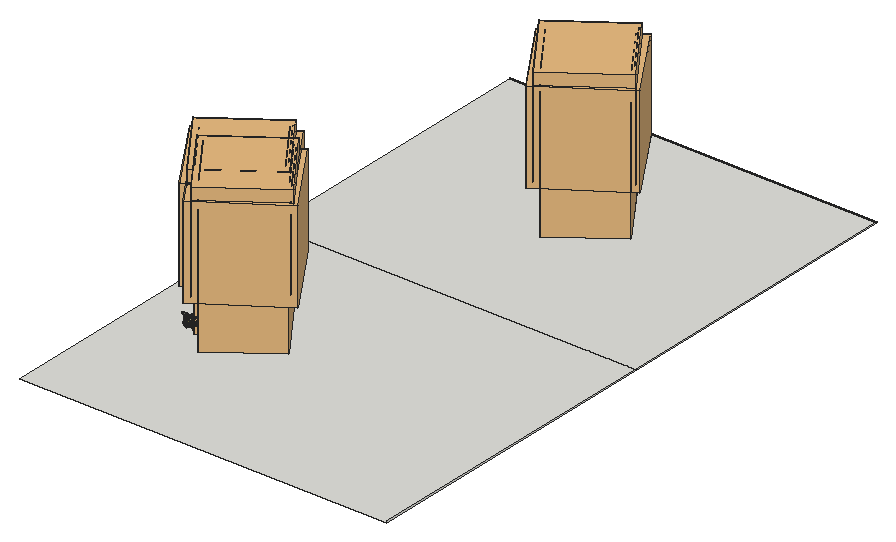
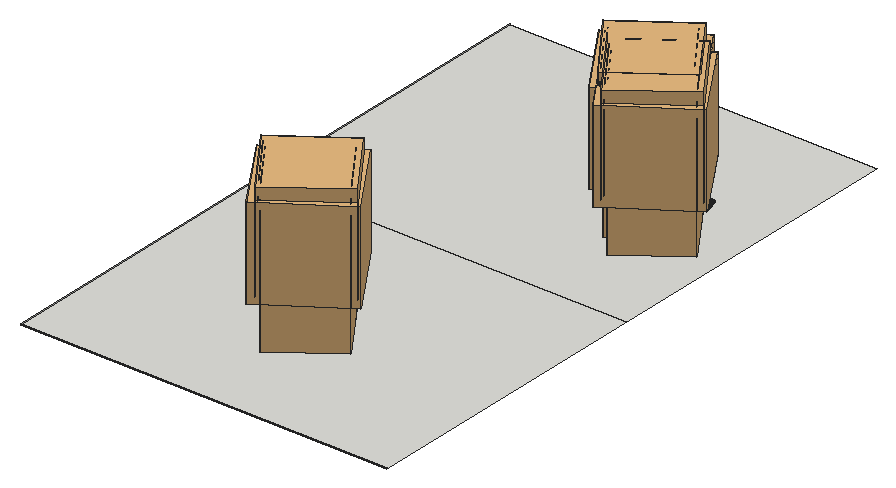
# SketchUp Ruby script. Lengths in inches.
U = 1.inch
M = Sketchup.active_model
def pt(a) = Geom::Point3d.new(a.map { |v| v * U })
def face(e, loops, mat)
  f = e.add_face(loops[0].map { |a| pt(a) })
  loops[1..].each { |l| e.add_face(l.map { |a| pt(a) }).erase! }
  f.material = f.back_material = mat if mat
  f
end
# faces: each face lists its corners as indices into pts; further lists are holes
def faces(e, pts, list, mat = nil) = list.each { |f| face(e, (f[0].is_a?(Array) ? f : [f]).map { |l| l.map { |i| pts[i] } }, mat) }
# xy, xz, yz: faces in a plane at the given z, y or x. An outline is a flat list of corners, or four numbers for a rectangle; further outlines are holes
def ring(l) = l.size == 4 ? [[l[0], l[1]], [l[2], l[1]], [l[2], l[3]], [l[0], l[3]]] : l.each_slice(2).to_a
def flat(e, list, mat, &to3) = list.each { |f| face(e, (f[0].is_a?(Array) ? f : [f]).map { |l| ring(l).map { |u, v| to3.(u, v) } }, mat) }
def xy(e, z, list, mat = nil) = flat(e, list, mat) { |x, y| [x, y, z] }
def xz(e, y, list, mat = nil) = flat(e, list, mat) { |x, z| [x, y, z] }
def yz(e, x, list, mat = nil) = flat(e, list, mat) { |y, z| [x, y, z] }
def lines(e, pts, list) = list.each { |a, b| e.add_line(pt(pts[a]), pt(pts[b])) }
# prism: a flat outline (further loops are holes) pulled along v
def prism(e, loops, v, mat = nil)
  f = face(e, loops, mat); d = Geom::Vector3d.new(v.map { |x| x * U })
  f.pushpull(f.normal.samedirection?(d) ? d.length : -d.length)
end
def box(e, o, s, mat = nil) = prism(e, [[o, [o[0] + s[0], o[1], o[2]], [o[0] + s[0], o[1] + s[1], o[2]], [o[0], o[1] + s[1], o[2]]]], [0, 0, s[2]], mat)
def at(x, y, z, deg = 0) = Geom::Transformation.translation(pt([x, y, z])) * Geom::Transformation.rotation(ORIGIN, Z_AXIS, deg.degrees)
def axes(o, x, y, z) = Geom::Transformation.new([*x, 0, *y, 0, *z, 0, *pt(o).to_a, 1])
def part(name) = M.definitions.add(name)
# library, detail: a bought-in or finely detailed component or shape, given as its bounding box
def library(name, o, s) = part(name).tap { |d| box(d.entities, o, s) }
def detail(e, o, s) = box(e.add_group.entities, o, s)
def put(e, d, t, mat = nil) = e.add_instance(d, t).tap { |i| i.material = mat if mat }
def group(e, t, mat = nil) = e.add_group.tap { |g| g.transformation = t; g.material = mat if mat }.entities
root = M.entities
M.materials.add("028_190k_fullGeometry_Material \#4").color = [120, 148, 64]
M.materials.add("Colorsadfasdfa0sd1f06w3").color = [153, 130, 61]
M.materials.add("Euphorbia asdfasd0f150160s159w").color = [180, 173, 131]
M.materials.add("Euphorbiaasdfa0sdf1a56sd016wow Leaf SU").color = [141, 134, 72]
M.materials.add("asdfasdf0165f6asdLeafVar1sfd015as60f1as6").color = [231, 235, 211]
M.materials.add("dw_stemssadfasdfa0sdf1s01d6w1").color = [90, 97, 50]
M.materials.add("viburnumblaasdfas0df1w06d").color = [98, 102, 84]
M.materials.add("viburnumbladsadfasdfad0w122").color = [125, 129, 119]
c1 = part("Component\#315")
p = [[0.25,0,0],[2.05,0.01,0.35],[1.81,4.2,1.66],[0,4.19,1.3125]]
faces(c1.entities,p,[[0,1,2,3]],"viburnumbladsadfasdfad0w122")
c2 = part("viburnumblad2")
put(c2.entities,c1,axes([-19.23,-4.49,-32.18],[83.35428,0,0],[0,79.38502,0],[0,0,83.35428]))
c3 = part("Component\#314")
p = [[0.14,0,0],[2.58,0.05,0.25],[2.44,5.11,2.64],[0,5.05,2.39]]
faces(c3.entities,p,[[0,1,2,3]],"viburnumblaasdfas0df1w06d")
c4 = part("viburnumblad1\#2")
put(c4.entities,c3,axes([-37.25,6.23,19.31],[75.98784,0,0],[0,65.50676,0],[0,0,75.98784]))
c5 = part("vdw_leaf\#3")
p = [[0,0,0],[-2.77,1.61,2.32],[-4.3125,6.1,4.5],[-3.97,13.49,6.09],[-2.47,18.57,6.3],[-0.2,22.73,5.75],
  [2.54,19.66,6.85],[4.3,15.93,7.09],[5.03,7.6,5.43],[3.32,1.76,2.74]]
faces(c5.entities,p,[[0,1,2,3,4,5],[0,5,6,7,8,9]],"asdfasdf0165f6asdLeafVar1sfd015as60f1as6")
c6 = part("dw_brancj_2\#2")
p = [[9.7,-0.22,29.95],[0.23,-1.96,0.34],[-0.05,1.51,0.11],[9.65,1.51,29.46],[18.64,-8.75,84.43],[18.96,-6.63,84.625],
  [1.53,6.02,63.68],[1.42,8.18,63.25],[-10.58,8.77,161.17],[-10.41,9.98,160.68],[26.34,-9.37,211.72],[26.57,-8.28,211.23]]
faces(c6.entities,p,[[0,1,2],[0,2,3],[4,0,3],[4,3,5],[6,0,3],[6,3,7],[8,6,7],[8,7,9],
  [10,4,5],[10,5,11]],"dw_stemssadfasdfa0sdf1s01d6w1")
c7 = part("vdw_branch2\#3")
put(c7.entities,c5,axes([19.53,-5.9,102.42],[1.12377,-0.50004,0],[0.46097,1.03596,0.47664],[-0.19377,-0.43548,1.13389]))
put(c7.entities,c5,axes([-5.89,6.52,109.44],[-1.07209,0.83679,0],[-0.77141,-0.98832,0.52702],[0.32427,0.41545,1.25373]))
put(c7.entities,c5,axes([-0.44,8.23,75.28],[0.88709,-0.9947,0],[0.92159,0.82189,0.33087],[-0.25219,-0.22491,1.26111]))
put(c7.entities,c5,axes([24.71,-8.97,190.81],[-0.82641,0.91101,0],[-0.83983,-0.76184,0.47664],[0.35303,0.32025,1.13389]))
put(c7.entities,c5,axes([-2.29,8.24,91.35],[1.24603,-0.47303,0],[0.43826,1.15445,0.33087],[-0.11993,-0.31592,1.26111]))
put(c7.entities,c5,axes([12.26,-3.11,37.92],[-0.64625,1.02205,0.22511],[-1.04383,-0.61044,-0.22511],[-0.07533,-0.30931,1.18809]))
put(c7.entities,c5,axes([26.17,-9.17,210.27],[-0.99452,-0.10453,0],[0.09636,-0.91681,0.38752],[-0.04051,0.38539,0.92186]))
put(c7.entities,c5,axes([-6.07,9.4,125.35],[-0.90214,-0.98107,0],[0.90896,-0.83583,0.33087],[-0.24874,0.22873,1.26111]))
put(c7.entities,c5,axes([-4.13,7.29,110.58],[0.44715,-1.078,0.64369],[1.05816,0.63649,0.33087],[-0.58725,0.40856,1.09216]))
put(c7.entities,c5,axes([23.91,-8.22,171.96],[0.62307,0.85009,-0.63406],[-0.71531,0.8798,0.47664],[0.78296,0.12729,0.94004]))
put(c7.entities,c6,at(-0.09,0.18,-0.25),"dw_stemssadfasdfa0sdf1s01d6w1")
put(c7.entities,c5,axes([23.34,-9.65,156.59],[-0.31364,-1.00782,0.58216],[1.10369,-0.17062,0.29925],[-0.17137,0.6239,0.98776]))
put(c7.entities,c5,axes([15.03,-3.37,58.83],[-1.05425,-0.00194,0.58442],[-0.14303,-1.11707,-0.26172],[0.55355,-0.3046,0.99755]))
put(c7.entities,c5,axes([-11.625,9.46,160.37],[0.36812,0.92978,0],[-0.85713,0.33936,0.38752],[0.3603,-0.14265,0.92186]))
put(c7.entities,c5,axes([21.32,-8.53,138.72],[1.21379,0.19904,0],[-0.19904,1.21379,0],[0,0,1.23]))
put(c7.entities,c5,axes([22.54,-9.2,141.43],[-1.02887,0.17955,0.60182],[-0.23387,-1.13057,-0.06253],[0.56696,-0.17376,1.02111]))
put(c7.entities,c5,axes([23.9,-8.82,173.84],[-1.14567,-0.37474,0],[0.35918,-1.0981,0.04438],[-0.01409,0.04308,1.17993]))
put(c7.entities,c5,axes([-7.84,8.92,143.59],[-1.26971,0.40522,0],[-0.37543,-1.17638,0.33087],[0.10274,0.32192,1.26111]))
put(c7.entities,c5,axes([19.77,-8.01,85.98],[-0.32405,-1.14591,0.18674],[1.10278,-0.32969,-0.10948],[0.15845,0.14442,1.16117]))
put(c7.entities,c5,axes([-0.62,5.76,76.34],[-0.08879,1.17576,-0.67771],[-1.34525,-0.16582,-0.11144],[-0.17897,0.66309,1.17383]))
put(c7.entities,c5,axes([20.49,-8.22,121.07],[0.39924,-0.78471,-0.8233],[1.08735,0.33121,0.2116],[0.09035,-0.83005,0.83495]))
put(c7.entities,c5,axes([15.15,-3.72,62.9],[1.16251,0.40128,-0.0211],[-0.39924,1.16074,0.07874],[0.0456,-0.06757,1.2273]))
put(c7.entities,c5,axes([20.72,-8.08,120.26],[-0.03693,1.2277,-0.06551],[-1.22944,-0.03698,0],[-0.00197,0.06548,1.22825]))
put(c7.entities,c5,axes([22.58,-8.36,155.57],[-0.56247,1.09386,0],[-1.00839,-0.51852,0.47664],[0.42389,0.21796,1.13389]))
put(c7.entities,c5,axes([3.97,3.13,57.96],[-1.09459,0.76041,0],[-0.72262,-1.0402,-0.1735],[-0.10109,-0.14552,1.29352]))
put(c7.entities,c5,axes([-10.8,9.06,160.75],[-0.66334,-0.72138,0],[0.66835,-0.61458,0.24329],[-0.1829,0.16818,0.92729]))
put(c7.entities,c5,axes([19.06,-9.3125,103.96],[-1.01345,0.25553,-0.60051],[-0.2265,-1.12952,-0.09839],[-0.59598,0.03076,1.01889]))
put(c7.entities,c5,axes([18.07,-6.2,81.7],[-0.56247,1.09386,0],[-1.00839,-0.51852,0.47664],[0.42389,0.21796,1.13389]))
put(c7.entities,c5,axes([12.95,-0.39,43.31],[0.13044,-1.19832,0],[1.11025,0.12085,0.29925],[-0.30382,-0.03307,1.14057]))
put(c7.entities,c5,axes([2.28,8.28,56.18],[1.32413,-0.31027,0],[0.30923,1.31968,-0.11144],[0.02542,0.1085,1.35543]))
put(c7.entities,c5,axes([-7.55,9.96,143.07],[1.34251,-0.21744,0],[0.20045,1.23761,0.52702],[-0.08426,-0.52024,1.25373]))
put(c7.entities,c5,axes([26.15,-8.25,210.66],[0.94661,-0.25364,0],[0.235,0.87703,0.24329],[-0.06431,-0.24,0.92729]))
put(c7.entities,c5,axes([-6.48,11.37,125.16],[0.64635,1.10315,0.46356],[-1.16569,0.46153,0.52702],[0.27017,-0.6478,1.16488]))
put(c7.entities,c5,axes([25.74,-8.35,191.28],[0.13044,-1.19832,0],[1.11025,0.12085,0.29925],[-0.30382,-0.03307,1.14057]))
put(c7.entities,c5,axes([-5.125,7.47,91.6],[-1.10024,0.63688,0.48318],[-0.78682,-1.00808,-0.46292],[0.14137,-0.65404,1.184]))
c8 = part("Component\#306")
p = [[4.55,0.11,0],[4.55,0,0],[2.84,0,3.13],[2.84,0.11,3.13],[4.625,0.05,0.04],[2.92,0.05,3.15],
  [2.08,0,8.07],[2.08,0.11,8.07],[2.16,0.05,8.1],[0,0,12.54],[0,0.11,12.54],[0.07,0.05,12.58]]
faces(c8.entities,p,[[0,1,2,3],[1,4,5,2],[1,0,4],[4,0,3,5],[3,2,6,7],[2,5,8,6],[5,3,7,8],[7,6,9,10],
  [6,8,11,9],[8,7,10,11],[10,9,11]],"Colorsadfasdfa0sd1f06w3")
c9 = part("Component\#301")
xy(c9.entities,0,[[0,0,0.7,3.1]],"Euphorbiaasdfa0sdf1a56sd016wow Leaf SU")
c10 = part("Leaf rosette")
put(c10.entities,c9,axes([2.21,1.74,0.13],[-0.4441,0.47879,-0.0956],[-0.4878,-0.4406,0.05935],[-0.03146,0.16757,0.98536]))
put(c10.entities,c9,axes([2.29,1.9,0.17],[-0.62678,-0.10063,-0.18061],[0.01105,-0.59203,0.2915],[-0.31282,0.41486,0.85442]))
put(c10.entities,c9,axes([2.09,1.69,0.1],[-0.10438,0.65169,0],[-0.65169,-0.10438,0],[0,0,1]))
put(c10.entities,c9,axes([1.97,1.77,0.02],[0.31114,0.5228,0.25587],[-0.57125,0.32993,0.02052],[-0.16918,-0.3502,0.92127]))
put(c10.entities,c9,axes([1.93,1.95,0],[0.54816,-0.03215,0.36617],[-0.11878,0.60671,0.23108],[-0.52706,-0.39065,0.75472]))
put(c10.entities,c9,axes([2.04,2.1,0.05],[0.26275,-0.55867,0.23335],[0.34186,0.34684,0.44545],[-0.75711,-0.08556,0.64766]))
put(c10.entities,c9,axes([2.22,2.08,0.13],[-0.29265,-0.59104,-0.02512],[0.40323,-0.2198,0.47401],[-0.65583,0.2952,0.69479]))
c11 = part("Component\#308")
xy(c11.entities,0,[[0,0,5.01,4.64]],"Euphorbia asdfasd0f150160s159w")
c12 = part("Component\#316")
put(c12.entities,c8,at(2.35,3.5,0))
put(c12.entities,c10,at(0.25,1.59,12.45))
put(c12.entities,c11,axes([7.46,0.77,3.64],[0.10848,0.99337,0.03799],[-0.82378,0.11122,-0.55589],[-0.55643,0.02901,0.83038]))
put(c12.entities,c11,axes([1.97,2.58,1.93],[0.80762,-0.50565,0.30344],[0.47433,0.86274,0.17519],[-0.35038,0.00244,0.93661]))
put(c12.entities,c11,axes([5.79,0.14,3.9],[0.5013,0.78918,0.35482],[-0.74775,0.60146,-0.2813],[-0.4354,-0.1243,0.89162]))
put(c12.entities,c11,axes([1.87,2.6,3.75],[0.73154,-0.49698,0.46676],[0.47433,0.86274,0.17519],[-0.48976,0.09324,0.86686]))
put(c12.entities,c11,axes([3.91,7.06,6.66],[-0.50827,-0.83837,-0.19699],[0.8278,-0.53869,0.15675],[-0.23753,-0.08339,0.96779]))
put(c12.entities,c11,axes([1.2,3.99,6.83],[0.56066,-0.79708,0.22433],[0.74237,0.60386,0.29025],[-0.36682,0.0038,0.93028]))
put(c12.entities,c9,axes([2.42,3.73,12.57],[-0.1322,-0.64472,0.04955],[0.10064,0.02944,0.65162],[-0.9678,0.2092,0.14002]))
put(c12.entities,c9,axes([2.57,3.43,12.63],[-0.62833,0.089,-0.18134],[-0.19954,-0.36568,0.51192],[-0.04764,0.82148,0.56824]))
put(c12.entities,c11,axes([4.04,6.92,11.09],[-0.67411,-0.5063,-0.5378],[0.44628,-0.85937,0.24964],[-0.58857,-0.07172,0.80526]))
put(c12.entities,c9,axes([2.5,3.49,12.74],[-0.62833,0.089,-0.18134],[-0.18746,-0.03618,0.63178],[0.11402,0.98935,0.09049]))
put(c12.entities,c9,axes([2.3,3.27,12.51],[0.02916,0.64747,0.12464],[-0.56235,-0.04072,0.34308],[0.5216,-0.18387,0.83314]))
put(c12.entities,c11,axes([0.26,4.96,9.69],[0.33661,-0.92735,0.16343],[0.73504,0.36725,0.56995],[-0.58857,-0.07172,0.80526]))
put(c12.entities,c11,axes([4.76,6.31,12.62],[-0.95056,-0.1129,-0.28929],[0.09021,-0.99179,0.09066],[-0.29715,0.06008,0.95294]))
put(c12.entities,c11,axes([5.2,6.55,10.37],[-0.76372,-0.27738,-0.58291],[0.26517,-0.95808,0.10848],[-0.58857,-0.07172,0.80526]))
c13 = part("Plant stem")
p = [[2.84,0.11,3.13],[2.84,0,3.13],[2.08,0,8.07],[2.08,0.11,8.07],[2.92,0.05,3.15],[2.16,0.05,8.1],
  [0,0,12.54],[0,0.11,12.54],[0.07,0.05,12.58]]
faces(c13.entities,p,[[0,1,2,3],[1,4,5,2],[4,0,3,5],[3,2,6,7],[2,5,8,6],[5,3,7,8],[7,6,8]],"Colorsadfasdfa0sd1f06w3")
c14 = part("Leafy shoot")
put(c14.entities,c13,at(2.35,3.5,0))
put(c14.entities,c10,at(0.25,1.59,12.45))
put(c14.entities,c11,axes([1.87,2.6,3.75],[0.73154,-0.49698,0.46676],[0.47433,0.86274,0.17519],[-0.48976,0.09324,0.86686]))
put(c14.entities,c11,axes([3.91,7.06,6.66],[-0.50827,-0.83837,-0.19699],[0.8278,-0.53869,0.15675],[-0.23753,-0.08339,0.96779]))
put(c14.entities,c11,axes([1.2,3.99,6.83],[0.56066,-0.79708,0.22433],[0.74237,0.60386,0.29025],[-0.36682,0.0038,0.93028]))
put(c14.entities,c9,axes([2.42,3.73,12.57],[-0.1322,-0.64472,0.04955],[0.10064,0.02944,0.65162],[-0.9678,0.2092,0.14002]))
put(c14.entities,c9,axes([2.57,3.43,12.63],[-0.62833,0.089,-0.18134],[-0.19954,-0.36568,0.51192],[-0.04764,0.82148,0.56824]))
put(c14.entities,c11,axes([4.04,6.92,11.09],[-0.67411,-0.5063,-0.5378],[0.44628,-0.85937,0.24964],[-0.58857,-0.07172,0.80526]))
put(c14.entities,c9,axes([2.5,3.49,12.74],[-0.62833,0.089,-0.18134],[-0.18746,-0.03618,0.63178],[0.11402,0.98935,0.09049]))
put(c14.entities,c9,axes([2.3,3.27,12.51],[0.02916,0.64747,0.12464],[-0.56235,-0.04072,0.34308],[0.5216,-0.18387,0.83314]))
put(c14.entities,c11,axes([0.26,4.96,9.69],[0.33661,-0.92735,0.16343],[0.73504,0.36725,0.56995],[-0.58857,-0.07172,0.80526]))
put(c14.entities,c11,axes([4.76,6.31,12.62],[-0.95056,-0.1129,-0.28929],[0.09021,-0.99179,0.09066],[-0.29715,0.06008,0.95294]))
put(c14.entities,c11,axes([5.2,6.55,10.37],[-0.76372,-0.27738,-0.58291],[0.26517,-0.95808,0.10848],[-0.58857,-0.07172,0.80526]))
put(c14.entities,c11,axes([7.03,0.77,3.77],[0.19714,0.84663,0.32426],[-0.94994,0.28899,-0.30484],[-0.2731,-0.45173,0.91532]))
c15 = part("Groundcover plant")
put(c15.entities,c12,axes([0.82,1.83,0.8125],[0.98541,0,-0.17021],[0,1,0],[0.17021,0,0.98541]))
put(c15.entities,c14,axes([4.45,-0.84,-2.24],[0.69527,0.50616,0],[-0.50264,0.69042,-0.10135],[-0.05965,0.08194,0.85401]))
put(c15.entities,c14,axes([1.85,7.37,-3.38],[0.7038,-0.47341,0.14191],[0.46407,0.71797,0.09357],[-0.16999,0,0.84303]))
put(c15.entities,c14,axes([6.9,-3.65,-2.52],[0.79351,0.57769,0],[-0.57366,0.78798,-0.11567],[-0.06808,0.09351,0.97468]))
put(c15.entities,c14,axes([1.36,5.18,-2.66],[0.50674,-0.34086,0.10218],[0.33413,0.51694,0.06737],[-0.12239,0,0.60698]))
put(c15.entities,c14,axes([5.76,-1.49,-2.17],[0.43479,0.43181,0.07251],[-0.43488,0.43544,-0.06951],[-0.06212,-0.06169,0.61918]))
c16 = part("Groundcover clump")
put(c16.entities,c15,axes([25.06,6.72,0.82],[-0.74291,1.22188,0],[-1.22188,-0.74291,0],[0,0,1]))
put(c16.entities,c15,axes([-0.76,2.1875,0.82],[1.43,0,0],[0,1.43,0],[0,0,1]))
put(c16.entities,c15,axes([8.21,24.79,0.82],[-0.6403,-1.27864,0],[1.27864,-0.6403,0],[0,0,1]))
c17 = library("028_190k_fullGeometry_0",[-319.99,-281.1,-2.15],[577.33,562.38,1159.36])
c18 = library("028_190k_fullGeometry_1",[-333.4,-281.7,421.48],[600.33,578.53,738.83])
c19 = library("028_190k_fullGeometry_2",[-3584003,-3264710,4041818.25],[6566285.5,6460741.75,7903602.75])
c20 = library("028_190k_fullGeometry_3",[-353.86,-324.57,405.22],[652.24,636.69,781.83])
c21 = part("028_190k_fullGeometry_4")
p = [[125.51,152.8,882.93],[125.36,152.82,883.01],[124.8,155.5625,881.05]]
faces(c21.entities,p,[[0,1,2]],"028_190k_fullGeometry_Material \#4")
c22 = part("028_190k_fullGeometry")
g1 = group(c22.entities,at(0,0,0))
put(g1,c17,axes([0,0,0],[0.18998,-0.26642,0],[0.26642,0.18998,0],[0,0,0.32722]))
put(g1,c18,axes([0,0,0],[0.18998,-0.26642,0],[0.26642,0.18998,0],[0,0,0.32722]))
put(g1,c19,axes([0,0,0],[0.00002,-0.00003,0],[0.00003,0.00002,0],[0,0,0.00003]))
put(g1,c20,axes([0,0,0],[0.18998,-0.26642,0],[0.26642,0.18998,0],[0,0,0.32722]))
put(g1,c21,axes([0,0,0],[0.18998,-0.26642,0],[0.26642,0.18998,0],[0,0,0.32722]))
xy(root,-9,[[2076.625,0,3026.5,807.5],[2076.625,807.5,3026.5,1583.3125]])
xz(root,1583.3125,[[2076.625,-9,3026.5,-6]])
yz(root,3026.5,[[0,-9,807.5,-6],[807.5,-9,1583.3125,-6]])
put(root,c2,axes([2215.15,362.91,28.11],[-0.00284,-0.00899,0.01128],[0.01228,-0.00546,-0.00125],[0.00539,0.01,0.00933]))
put(root,c2,axes([2213.87,361.91,27.32],[0.00722,-0.01189,0.00649],[0.01053,0.00219,-0.0077],[0.0056,0.00897,0.01021]))
put(root,c4,axes([2211.54,359.55,25.5],[0.01385,-0.00786,0.00256],[0.00839,0.01058,-0.01294],[0.00399,0.01072,0.01136]))
put(root,c2,axes([2208.15,362.49,28.56],[-0.01171,0.00153,-0.0034],[-0.00332,-0.0036,0.00923],[0.00008,0.01052,0.00323]))
put(root,c2,axes([2207.59,363.09,27.32],[-0.00352,-0.00505,0.00939],[0.01197,-0.00026,0.00408],[-0.00173,0.01006,0.00403]))
put(root,c2,axes([2213.35,360.82,28.75],[0.01049,0.00127,-0.00935],[-0.00649,0.01342,-0.00547],[0.00778,0.00774,0.00978]))
put(root,c2,axes([2206.95,362.34,28.96],[0.00325,0.00384,-0.00943],[-0.01118,0.00267,-0.00269],[0.00139,0.01021,0.00373]))
put(root,c2,axes([2208.18,364.125,28.21],[-0.01052,-0.00268,0.00462],[0.00552,-0.00368,0.01018],[-0.00102,0.01046,0.0033]))
put(root,c2,axes([2207.85,363.48,29.39],[-0.00534,0.00476,-0.00922],[-0.00963,-0.00133,0.0047],[0.00092,0.0102,0.00386]))
put(root,c2,axes([2213.94,362.66,29.32],[0.01262,-0.00712,-0.00249],[0.00385,0.01054,-0.01059],[0.00659,0.00804,0.0104]))
put(root,c2,axes([2215.34,364.32,29.63],[0.00691,-0.01139,0.00621],[0.0117,0.00243,-0.00856],[0.0056,0.00897,0.01021]))
put(root,c7,axes([2239.84,354.51,6.3],[0.0097,0.14118,-0.10053],[-0.16302,0.01121,0],[0.0056,0.08151,0.17413]))
put(root,c2,axes([2206.95,364.36,27.76],[0.00534,-0.00476,0.00922],[0.0104,0.00387,-0.00404],[-0.00165,0.00955,0.00498]))
put(root,c2,axes([2206.27,363.72,28.9375],[0.01052,0.00268,-0.00462],[-0.0054,0.00599,-0.0087],[0.00028,0.0093,0.00555]))
put(root,c2,axes([2207.82,365.66,28.31],[-0.00367,-0.00526,0.00978],[0.01109,-0.00025,0.00378],[-0.00173,0.01006,0.00403]))
put(root,c2,axes([2214.72,363.35,31.09],[0.01093,0.00132,-0.00974],[-0.00601,0.01242,-0.00506],[0.00778,0.00774,0.00978]))
put(root,c2,axes([2206.84,364.77,29.93],[0.00367,0.00526,-0.00978],[-0.01118,0.00267,-0.00269],[0.001,0.0097,0.00482]))
put(root,c16,axes([2211.35,348.19,7.84],[1.49047,0,0],[0,1.49047,0],[0,0,1.49047]))
put(root,c2,axes([2206.4,365.42,28.68],[0.01122,-0.00147,0.00326],[0.00359,0.00643,-0.00917],[-0.00081,0.00924,0.00561]))
put(root,c22,at(2316.2,429.9,-5.3))
put(root,c22,at(2264.3,482.58,-5.3))
put(root,c22,at(2560.7,1232.38,-5.3))
